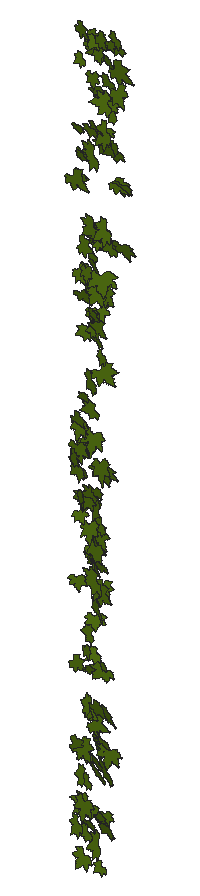
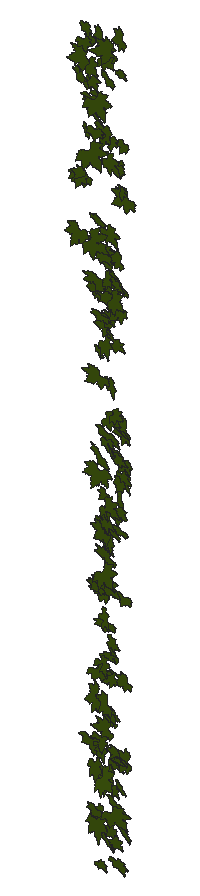
# SketchUp Ruby script. Lengths in inches.
U = 1.inch
M = Sketchup.active_model
def pt(a) = Geom::Point3d.new(a.map { |v| v * U })
def face(e, loops, mat)
  f = e.add_face(loops[0].map { |a| pt(a) })
  loops[1..].each { |l| e.add_face(l.map { |a| pt(a) }).erase! }
  f.material = f.back_material = mat if mat
  f
end
# faces: each face lists its corners as indices into pts; further lists are holes
def faces(e, pts, list, mat = nil) = list.each { |f| face(e, (f[0].is_a?(Array) ? f : [f]).map { |l| l.map { |i| pts[i] } }, mat) }
# xy, xz, yz: faces in a plane at the given z, y or x. An outline is a flat list of corners, or four numbers for a rectangle; further outlines are holes
def ring(l) = l.size == 4 ? [[l[0], l[1]], [l[2], l[1]], [l[2], l[3]], [l[0], l[3]]] : l.each_slice(2).to_a
def flat(e, list, mat, &to3) = list.each { |f| face(e, (f[0].is_a?(Array) ? f : [f]).map { |l| ring(l).map { |u, v| to3.(u, v) } }, mat) }
def xy(e, z, list, mat = nil) = flat(e, list, mat) { |x, y| [x, y, z] }
def xz(e, y, list, mat = nil) = flat(e, list, mat) { |x, z| [x, y, z] }
def yz(e, x, list, mat = nil) = flat(e, list, mat) { |y, z| [x, y, z] }
def lines(e, pts, list) = list.each { |a, b| e.add_line(pt(pts[a]), pt(pts[b])) }
# prism: a flat outline (further loops are holes) pulled along v
def prism(e, loops, v, mat = nil)
  f = face(e, loops, mat); d = Geom::Vector3d.new(v.map { |x| x * U })
  f.pushpull(f.normal.samedirection?(d) ? d.length : -d.length)
end
def box(e, o, s, mat = nil) = prism(e, [[o, [o[0] + s[0], o[1], o[2]], [o[0] + s[0], o[1] + s[1], o[2]], [o[0], o[1] + s[1], o[2]]]], [0, 0, s[2]], mat)
def at(x, y, z, deg = 0) = Geom::Transformation.translation(pt([x, y, z])) * Geom::Transformation.rotation(ORIGIN, Z_AXIS, deg.degrees)
def axes(o, x, y, z) = Geom::Transformation.new([*x, 0, *y, 0, *z, 0, *pt(o).to_a, 1])
def part(name) = M.definitions.add(name)
# library, detail: a bought-in or finely detailed component or shape, given as its bounding box
def library(name, o, s) = part(name).tap { |d| box(d.entities, o, s) }
def detail(e, o, s) = box(e.add_group.entities, o, s)
def put(e, d, t, mat = nil) = e.add_instance(d, t).tap { |i| i.material = mat if mat }
def group(e, t, mat = nil) = e.add_group.tap { |g| g.transformation = t; g.material = mat if mat }.entities
root = M.entities
M.materials.add("[Vegetation Blur 03]").color = [83, 114, 18]
c1 = part("ivy")
xy(c1.entities,0,[[0.782,0,0.786,0,0.787,0.005,0.789,0.009,0.821,0.072,0.875,0.147,1.001,0.272,1.073,0.331,1.137,0.363,1.178,0.379,1.223,0.384,1.272,0.383,1.311,0.374,1.36,0.355,1.399,0.334,1.491,0.285,1.541,0.244,1.583,0.199,1.617,0.15,1.64,0.128,1.662,0.115,1.717,0.105,1.745,0.093,1.784,0.054,1.819,0.057,1.854,0.064,1.882,0.075,1.896,0.074,1.91,0.071,1.937,0.063,1.964,0.053,1.99,0.038,2.016,0.015,2.034,0.002,2.04,0,2.038,0.003,2.036,0.007,2.033,0.038,2.036,0.068,2.045,0.1,2.055,0.116,2.064,0.123,2.077,0.129,2.088,0.129,2.106,0.132,2.118,0.13,2.179,0.132,2.207,0.133,2.225,0.133,2.242,0.138,2.22,0.162,2.207,0.186,2.206,0.213,2.212,0.236,2.228,0.262,2.247,0.274,2.298,0.283,2.355,0.294,2.37,0.296,2.376,0.295,2.377,0.3,2.377,0.303,2.385,0.329,2.411,0.37,2.426,0.392,2.449,0.407,2.511,0.426,2.561,0.444,2.619,0.466,2.589,0.469,2.561,0.476,2.501,0.5,2.449,0.516,2.424,0.523,2.401,0.535,2.377,0.556,2.372,0.568,2.36,0.575,2.268,0.586,2.225,0.592,2.207,0.599,2.194,0.61,2.143,0.65,2.13,0.664,2.122,0.682,2.123,0.7,2.13,0.719,2.148,0.75,2.17,0.781,2.195,0.807,2.221,0.828,2.284,0.874,2.291,0.88,2.288,0.887,2.276,0.9,2.267,0.916,2.265,0.933,2.273,0.967,2.292,1.002,2.313,1.03,2.334,1.054,2.348,1.067,2.358,1.074,2.363,1.076,2.362,1.081,2.35,1.094,2.347,1.11,2.35,1.143,2.359,1.18,2.385,1.254,2.415,1.324,2.448,1.393,2.45,1.4,2.446,1.398,2.44,1.394,2.427,1.383,2.402,1.36,2.376,1.339,2.345,1.324,2.305,1.309,2.282,1.303,2.273,1.306,2.245,1.294,2.212,1.287,2.187,1.291,2.163,1.301,2.142,1.316,2.134,1.327,2.124,1.325,2.09,1.292,2.053,1.259,2.014,1.234,1.973,1.215,1.954,1.21,1.931,1.208,1.909,1.212,1.893,1.22,1.879,1.233,1.872,1.248,1.867,1.281,1.864,1.319,1.821,1.258,1.773,1.197,1.726,1.141,1.698,1.121,1.679,1.116,1.666,1.117,1.647,1.122,1.632,1.129,1.62,1.141,1.617,1.154,1.617,1.219,1.621,1.254,1.623,1.268,1.623,1.281,1.618,1.314,1.606,1.346,1.603,1.375,1.607,1.403,1.603,1.467,1.599,1.499,1.605,1.525,1.614,1.552,1.629,1.577,1.635,1.589,1.629,1.587,1.618,1.582,1.596,1.566,1.581,1.556,1.568,1.552,1.557,1.55,1.545,1.553,1.531,1.562,1.522,1.572,1.504,1.591,1.486,1.611,1.474,1.631,1.457,1.666,1.455,1.684,1.457,1.698,1.452,1.715,1.444,1.728,1.424,1.754,1.419,1.772,1.423,1.786,1.434,1.819,1.444,1.848,1.446,1.855,1.44,1.861,1.43,1.867,1.386,1.904,1.349,1.948,1.326,1.973,1.31,1.995,1.288,2.048,1.284,2.153,1.287,2.254,1.284,2.255,1.282,2.253,1.278,2.247,1.274,2.237,1.266,2.216,1.226,2.125,1.208,2.076,1.184,2.033,1.155,1.984,1.135,1.942,1.111,1.899,1.083,1.861,1.053,1.85,1.059,1.83,1.061,1.809,1.056,1.79,1.049,1.767,1.04,1.749,1.018,1.733,0.994,1.726,0.942,1.734,0.95,1.6875,0.944,1.645,0.932,1.608,0.911,1.585,0.881,1.58,0.854,1.582,0.828,1.588,0.785,1.618,0.773,1.625,0.775,1.614,0.779,1.598,0.796,1.502,0.818,1.402,0.861,1.283,0.882,1.224,0.894,1.174,0.892,1.148,0.886,1.123,0.881,1.107,0.872,1.099,0.849,1.094,0.818,1.092,0.789,1.098,0.762,1.107,0.753,1.113,0.721,1.139,0.698,1.163,0.678,1.194,0.665,1.224,0.628,1.28,0.612,1.312,0.606,1.327,0.606,1.314,0.599,1.282,0.594,1.267,0.581,1.256,0.544,1.245,0.512,1.244,0.473,1.249,0.444,1.256,0.382,1.288,0.339,1.306,0.324,1.316,0.317,1.324,0.309,1.326,0.27,1.314,0.227,1.313,0.185,1.3125,0.152,1.317,0.122,1.328,0.092,1.345,0.073,1.353,0.079,1.338,0.092,1.308,0.117,1.249,0.13,1.215,0.139,1.164,0.147,1.148,0.157,1.136,0.163,1.122,0.174,1.086,0.177,1.067,0.182,1.054,0.186,1.043,0.191,1.038,0.211,1.028,0.237,1.005,0.25,0.974,0.253,0.96,0.25,0.944,0.242,0.914,0.243,0.906,0.249,0.902,0.26,0.894,0.289,0.88,0.307,0.873,0.322,0.862,0.364,0.799,0.403,0.738,0.431,0.709,0.439,0.691,0.441,0.678,0.4375,0.66,0.428,0.645,0.394,0.623,0.303,0.594,0.255,0.581,0.214,0.577,0.179,0.573,0.173,0.568,0.175,0.561,0.167,0.55,0.141,0.523,0.113,0.503,0.077,0.49,0.045,0.486,0.026,0.485,0.019,0.486,0.011,0.483,0,0.471,0.014,0.467,0.044,0.455,0.058,0.447,0.07,0.438,0.097,0.411,0.125,0.394,0.158,0.377,0.174,0.366,0.182,0.359,0.185,0.361,0.242,0.331,0.253,0.316,0.258,0.303,0.262,0.283,0.274,0.278,0.308,0.274,0.341,0.252,0.366,0.226,0.366,0.222,0.37,0.22,0.38,0.221,0.395,0.221,0.425,0.216,0.45,0.207,0.465,0.192,0.473,0.178,0.484,0.15,0.489,0.116,0.483,0.089,0.468,0.058,0.45,0.035,0.435,0.018,0.429,0.011,0.434,0.012,0.438,0.014,0.469,0.019,0.542,0.016,0.581,0.015,0.612,0.027,0.68,0.055,0.696,0.057,0.712,0.052,0.73,0.045,0.741,0.036,0.766,0.014]])
p = [[86.74,174.5,94.56],[86.66,174.5,94.56]]
lines(root,p,[[0,1]])
put(root,c1,axes([83.45,173.7,84.39],[0.11247,0.10768,-0.41349],[-0.50254,0.19726,-0.08297],[-0.08291,-1.04957,-0.05801]),"[Vegetation Blur 03]")
put(root,c1,axes([82.4,173.7,68.58],[0.38704,0.02073,0.09682],[0.11906,-0.06304,-0.31489],[0.00062,-0.83064,0.02631]),"[Vegetation Blur 03]")
put(root,c1,axes([82.79,173.7,75.08],[0.46711,-0.27655,-0.25561],[-0.31156,0.09667,-0.39569],[-0.13813,-1.15324,0.02812]),"[Vegetation Blur 03]")
put(root,c1,axes([82.6,173.7,91.86],[0.29162,-0.09248,0.04712],[0.06325,0.07335,-0.23812],[-0.03677,-0.60733,-0.03593]),"[Vegetation Blur 03]")
put(root,c1,axes([82.36,173.7,63.95],[0.20869,-0.00294,0.30527],[0.37402,-0.00987,-0.17032],[-0.00489,-0.88135,0.00089]),"[Vegetation Blur 03]")
put(root,c1,axes([82.53,173.7,74.5625],[0.11578,-0.07742,0.31422],[0.36947,-0.22297,-0.09932],[-0.11465,-0.79672,-0.00274]),"[Vegetation Blur 03]")
put(root,c1,axes([82.08,173.7,88.79],[0.38841,-0.03974,0.39058],[0.47889,0.01108,-0.31703],[-0.00798,-1.26829,-0.01501]),"[Vegetation Blur 03]")
put(root,c1,axes([82.88,173.7,89.65],[0.29613,-0.07388,-0.10232],[-0.12287,0.05638,-0.24327],[-0.04369,-0.65932,-0.00934]),"[Vegetation Blur 03]")
put(root,c1,axes([83.37,173.7,59.11],[0.14128,-0.20319,-0.29587],[-0.36071,0.14973,-0.1309],[-0.10517,-0.78653,0.05152]),"[Vegetation Blur 03]")
put(root,c1,axes([83.1,173.7,95.71],[0.23115,-0.1069,-0.165],[-0.20647,-0.0259,-0.19002],[-0.03067,-0.63139,0.03573]),"[Vegetation Blur 03]")
put(root,c1,axes([83.41,173.7,78.21],[0.08326,0.10722,-0.24971],[-0.31037,0.02564,-0.0672],[0.00148,-0.65202,-0.0437]),"[Vegetation Blur 03]")
put(root,c1,axes([82.8125,173.7,56.57],[0.42261,-0.28747,-0.1193],[-0.16204,-0.06467,-0.35783],[-0.12093,-0.91792,0.06257]),"[Vegetation Blur 03]")
put(root,c1,axes([82.48,173.7,59.61],[0.11289,-0.08937,0.40816],[0.50197,0.01041,-0.09212],[-0.00461,-1.05497,-0.03549]),"[Vegetation Blur 03]")
put(root,c1,axes([83.47,173.7,75.94],[0.13432,-0.12713,-0.31462],[-0.38869,0.03529,-0.11278],[-0.03669,-0.83931,0.04291]),"[Vegetation Blur 03]")
put(root,c1,axes([82.91,173.7,90.74],[0.29319,-0.08212,-0.05398],[-0.06371,0.04494,-0.24127],[-0.04367,-0.61685,-0.01039]),"[Vegetation Blur 03]")
put(root,c1,axes([82.6,173.7,71.81],[0.27283,0.0757,0.1916],[0.23721,-0.13013,-0.2169],[-0.01401,-0.72914,0.0586]),"[Vegetation Blur 03]")
put(root,c1,axes([82.38,173.7,75.48],[0.52424,-0.12738,0.15619],[0.18843,-0.07357,-0.4307],[-0.07036,-1.14606,0.01029]),"[Vegetation Blur 03]")
put(root,c1,axes([83.38,173.7,81.78],[0.19574,-0.01438,-0.25163],[-0.30815,-0.03945,-0.1593],[0.01245,-0.75048,0.0132]),"[Vegetation Blur 03]")
put(root,c1,axes([83.15,173.7,57.83],[0.47968,0.02946,-0.35016],[-0.4281,-0.06549,-0.39149],[0.03188,-1.32271,0.01158]),"[Vegetation Blur 03]")
put(root,c1,axes([83.65,173.7,84.9],[0.09556,-0.13792,-0.34176],[-0.41905,0.10501,-0.08471],[-0.06516,-0.87761,0.04357]),"[Vegetation Blur 03]")
put(root,c1,axes([82.79,173.7,74.375],[0.34163,-0.14558,0.05444],[0.07406,0.06471,-0.28235],[-0.063,-0.71335,-0.03672]),"[Vegetation Blur 03]")
put(root,c1,axes([82.59,173.7,84.14],[0.2559,0.03571,0.2999],[0.36108,-0.20047,-0.20147],[-0.07032,-0.89939,0.05682]),"[Vegetation Blur 03]")
put(root,c1,axes([83.25,173.7,60.26],[0.31122,-0.06083,-0.21678],[-0.26689,-0.02709,-0.25402],[-0.01391,-0.84152,0.02385]),"[Vegetation Blur 03]")
put(root,c1,axes([83.4,173.7,56.21],[0.24157,-0.07416,-0.2538],[-0.31175,0.01688,-0.19842],[-0.02861,-0.81014,0.0191]),"[Vegetation Blur 03]")
put(root,c1,axes([82.6,173.7,83.19],[0.40086,-0.0573,0.17483],[0.21594,0.13183,-0.32299],[0.00594,-0.92596,-0.0568]),"[Vegetation Blur 03]")
put(root,c1,axes([82.9,173.7,90.23],[0.11718,-0.12684,0.22641],[0.28293,-0.00575,-0.09804],[-0.02661,-0.61967,-0.04543]),"[Vegetation Blur 03]")
put(root,c1,axes([82.81,173.7,73.18],[0.52679,-0.06661,-0.07919],[-0.09633,0.02908,-0.43069],[-0.03439,-1.10187,-0.00658]),"[Vegetation Blur 03]")
put(root,c1,axes([82.7,173.7,76.92],[0.52102,-0.20474,0.04178],[0.03433,-0.18504,-0.42777],[-0.1065,-1.06132,0.06652]),"[Vegetation Blur 03]")
put(root,c1,axes([83.79,173.7,62.77],[0.05013,-0.17245,-0.31461],[-0.38087,0.18721,-0.05657],[-0.1028,-0.77773,0.05615]),"[Vegetation Blur 03]")
put(root,c1,axes([83,173.7,54.99],[0.48428,-0.17048,-0.13656],[-0.17611,-0.0992,-0.39652],[-0.06201,-1.04969,0.05965]),"[Vegetation Blur 03]")
put(root,c1,axes([82.49,173.7,76.59],[0.31137,-0.19726,0.4006],[0.48849,-0.13513,-0.26337],[-0.10722,-1.1885,-0.03655]),"[Vegetation Blur 03]")
put(root,c1,axes([83.89,173.7,59.78],[0.15704,0.2136,-0.46973],[-0.57168,0.3147,-0.1048],[-0.12334,-1.18664,-0.11235]),"[Vegetation Blur 03]")
put(root,c1,axes([83.49,173.7,58.8],[0.21308,-0.10262,-0.22404],[-0.27243,0.07685,-0.17812],[-0.0602,-0.71097,0.01308]),"[Vegetation Blur 03]")
put(root,c1,axes([83.8125,173.7,66.47],[0.09612,-0.08439,-0.33414],[-0.40558,0.12635,-0.08273],[-0.06933,-0.85613,0.02072]),"[Vegetation Blur 03]")
put(root,c1,axes([83.82,173.7,73.61],[0.20248,0.05039,-0.42079],[-0.51446,0.11243,-0.16277],[-0.042,-1.13431,-0.03483]),"[Vegetation Blur 03]")
put(root,c1,axes([82.9,173.7,85.32],[0.06821,0.02412,0.38984],[0.47536,-0.1037,-0.05439],[-0.04826,-0.98747,0.01524]),"[Vegetation Blur 03]")
put(root,c1,axes([82.76,173.7,96.75],[0.24867,-0.15858,0.33537],[0.40835,-0.11898,-0.21053],[-0.08971,-0.98119,-0.02867]),"[Vegetation Blur 03]")
put(root,c1,axes([83.82,173.7,77.97],[0.16222,0.03807,-0.33908],[-0.41557,-0.02093,-0.13279],[0.01621,-0.91758,-0.01104]),"[Vegetation Blur 03]")
put(root,c1,axes([82.57,173.7,59.83],[0.38921,-0.01895,0.37093],[0.44943,-0.16908,-0.31546],[-0.06835,-1.21968,0.03797]),"[Vegetation Blur 03]")
put(root,c1,axes([83.86,173.7,85.18],[0.08292,0.05054,-0.29306],[-0.34577,0.22171,-0.05915],[-0.09993,-0.72524,-0.0385]),"[Vegetation Blur 03]")
put(root,c1,axes([83.69,173.7,70.22],[0.33518,0.12814,-0.38098],[-0.46864,0.20726,-0.26366],[-0.04654,-1.16428,-0.08887]),"[Vegetation Blur 03]")
put(root,c1,axes([83.77,173.7,91.36],[0.33503,-0.17484,-0.44401],[-0.53885,0.1655,-0.28108],[-0.11328,-1.30432,0.02385]),"[Vegetation Blur 03]")
put(root,c1,axes([82.92,173.7,73.04],[0.31064,-0.27454,0.24989],[0.28954,-0.20759,-0.27561],[-0.1665,-0.87322,-0.01304]),"[Vegetation Blur 03]")
put(root,c1,axes([84.19,173.7,73.03],[0.10156,-0.07064,-0.4993],[-0.59327,0.30784,-0.08723],[-0.15326,-1.23847,0.0068]),"[Vegetation Blur 03]")
put(root,c1,axes([83.29,173.7,92.1],[0.37183,-0.05449,-0.06268],[-0.07386,0.08152,-0.30299],[-0.03383,-0.77703,-0.02739]),"[Vegetation Blur 03]")
put(root,c1,axes([83.92,173.7,69.5],[0.29364,-0.08887,-0.43973],[-0.53794,0.07502,-0.24166],[-0.05272,-1.26047,0.01662]),"[Vegetation Blur 03]")
put(root,c1,axes([83.3,173.7,61.67],[0.05383,0.00628,0.24765],[0.29967,-0.10102,-0.04299],[-0.04781,-0.62607,0.00942]),"[Vegetation Blur 03]")
put(root,c1,axes([83.78,173.7,86.52],[0.25146,0.10077,-0.27244],[-0.33679,0.12568,-0.19974],[-0.01997,-0.85077,-0.06178]),"[Vegetation Blur 03]")
put(root,c1,axes([83.6,173.7,87.57],[0.45075,-0.16208,-0.3284],[-0.40131,0.07789,-0.37294],[-0.08406,-1.24093,0.01948]),"[Vegetation Blur 03]")
put(root,c1,axes([82.9,173.7,57.62],[0.59208,-0.24793,0.06374],[0.06017,-0.19072,-0.48897],[-0.13036,-1.21404,0.0638]),"[Vegetation Blur 03]")
put(root,c1,axes([83.22,173.7,63.97],[0.19108,-0.09038,0.20852],[0.25839,0.11931,-0.14958],[0.021,-0.6456,-0.05683]),"[Vegetation Blur 03]")
put(root,c1,axes([83.13,173.7,84.73],[0.36627,-0.13941,0.12421],[0.13945,-0.15724,-0.30166],[-0.09113,-0.8009,0.0376]),"[Vegetation Blur 03]")
put(root,c1,axes([83.69,173.7,85.79],[0.23501,-0.07019,-0.1629],[-0.19555,0.08472,-0.19365],[-0.05258,-0.62881,-0.00791]),"[Vegetation Blur 03]")
put(root,c1,axes([83.2,173.7,65.14],[0.25479,-0.12423,0.18023],[0.21133,-0.13383,-0.2135],[-0.08804,-0.68079,0.00908]),"[Vegetation Blur 03]")
put(root,c1,axes([83.62,173.7,71.66],[0.37161,-0.21861,-0.25288],[-0.28876,0.23657,-0.31481],[-0.15463,-0.96714,-0.01984]),"[Vegetation Blur 03]")
put(root,c1,axes([83.25,173.7,56.28],[0.2775,-0.12673,0.11481],[0.14869,0.07236,-0.22682],[-0.03837,-0.63611,-0.04867]),"[Vegetation Blur 03]")
put(root,c1,axes([83.95,173.7,96.4],[0.21316,0.03069,-0.31446],[-0.38542,0.04396,-0.17335],[-0.01149,-0.90506,-0.01908]),"[Vegetation Blur 03]")
put(root,c1,axes([83.87,173.7,82.06],[0.16581,-0.12598,-0.20066],[-0.24842,0.03821,-0.1405],[-0.04988,-0.60905,0.03269]),"[Vegetation Blur 03]")
put(root,c1,axes([84.05,173.7,67.84],[0.20676,-0.07941,-0.38547],[-0.44776,0.31453,-0.17016],[-0.15519,-1.01328,-0.02261]),"[Vegetation Blur 03]")
put(root,c1,axes([83.78,173.7,81.8],[0.3273,-0.0909,-0.29956],[-0.34726,0.27044,-0.26563],[-0.12681,-0.97518,-0.04574]),"[Vegetation Blur 03]")
put(root,c1,axes([83.56,173.7,79.63],[0.43303,-0.27941,-0.22313],[-0.26455,0.14367,-0.37028],[-0.1523,-1.044,0.00876]),"[Vegetation Blur 03]")
put(root,c1,axes([83.47,173.7,59.71],[0.5589,-0.19272,-0.25961],[-0.28238,0.39595,-0.45114],[-0.17385,-1.26271,-0.10184]),"[Vegetation Blur 03]")
put(root,c1,axes([83.56,173.7,76.42],[0.33014,-0.06379,-0.05513],[-0.06679,0.02302,-0.2706],[-0.03261,-0.69306,-0.00391]),"[Vegetation Blur 03]")
put(root,c1,axes([83.44,173.7,61.71],[0.13106,0.04715,0.22271],[0.27208,-0.09295,-0.10355],[-0.03102,-0.61597,0.03267]),"[Vegetation Blur 03]")
put(root,c1,axes([83.42,173.7,82.65],[0.34203,-0.05341,0.04309],[0.05121,-0.04542,-0.27956],[-0.02898,-0.71072,0.01463]),"[Vegetation Blur 03]")
put(root,c1,axes([83.64,173.7,96.8125],[0.33694,0.0048,-0.1079],[-0.13035,-0.11296,-0.27192],[0.0222,-0.7362,0.04102]),"[Vegetation Blur 03]")
put(root,c1,axes([83.44,173.7,75.48],[0.09035,0.0602,0.28294],[0.33236,-0.23291,-0.06289],[-0.10289,-0.69949,0.04529]),"[Vegetation Blur 03]")
put(root,c1,axes([83.89,173.7,65.49],[0.26178,-0.07777,-0.19292],[-0.23918,-0.11506,-0.20887],[0.01,-0.71663,0.05447]),"[Vegetation Blur 03]")
put(root,c1,axes([83.14,173.7,71.55],[0.46252,-0.08041,0.20679],[0.23593,-0.28736,-0.36906],[-0.10033,-1.0465,0.08545]),"[Vegetation Blur 03]")
put(root,c1,axes([83.35,173.7,66.91],[0.41222,0.08825,0.09854],[0.12607,-0.1297,-0.333],[0.02291,-0.87434,0.05934]),"[Vegetation Blur 03]")
put(root,c1,axes([83.25,173.7,69.91],[0.09143,0.21564,0.47102],[0.58317,-0.16267,-0.06368],[-0.06308,-1.19139,0.09395]),"[Vegetation Blur 03]")
put(root,c1,axes([83.94,173.7,65.27],[0.3587,-0.08547,-0.26789],[-0.31864,0.17898,-0.29317],[-0.08908,-0.98439,-0.03004]),"[Vegetation Blur 03]")
put(root,c1,axes([83.69,173.7,84.04],[0.46854,-0.05722,-0.15501],[-0.19159,-0.07548,-0.38134],[-0.0119,-1.03762,0.03629]),"[Vegetation Blur 03]")
put(root,c1,axes([84.02,173.7,60.8],[0.31159,-0.10577,-0.25159],[-0.29051,0.23223,-0.255],[-0.11522,-0.87155,-0.03742]),"[Vegetation Blur 03]")
put(root,c1,axes([83.44,173.7,94.8],[0.3823,-0.12513,0.1329],[0.15394,-0.13225,-0.31454],[-0.08072,-0.8448,0.02956]),"[Vegetation Blur 03]")
put(root,c1,axes([83.24,173.7,95.86],[0.15219,-0.0035,0.49259],[0.60198,0.09401,-0.12377],[0.04388,-1.27745,-0.01046]),"[Vegetation Blur 03]")
put(root,c1,axes([83.59,173.7,82.125],[0.08947,-0.09548,0.30203],[0.3696,-0.08246,-0.07703],[-0.05008,-0.77914,-0.02886]),"[Vegetation Blur 03]")
put(root,c1,axes([84.17,173.7,56.15],[0.33567,-0.36714,-0.32626],[-0.40941,0.10373,-0.29893],[-0.15499,-1.06915,0.08303]),"[Vegetation Blur 03]")
put(root,c1,axes([83.98,173.7,94.33],[0.49914,0.06889,-0.35402],[-0.43405,0.1716,-0.40237],[-0.0297,-1.34994,-0.06922]),"[Vegetation Blur 03]")
put(root,c1,axes([83.26,173.7,76.58],[0.64177,-0.16774,0.0763],[0.07979,-0.21804,-0.52237],[-0.09498,-1.31665,0.07678]),"[Vegetation Blur 03]")
put(root,c1,axes([84.62,173.7,87.19],[0.20681,0.14961,-0.50522],[-0.62308,0.08477,-0.16594],[-0.01632,-1.34039,-0.06689]),"[Vegetation Blur 03]")
put(root,c1,axes([83.7,173.7,73.4],[0.23912,-0.07387,0.13682],[0.16931,0.00875,-0.19635],[-0.02693,-0.60087,-0.01968]),"[Vegetation Blur 03]")
put(root,c1,axes([83.46,173.7,60.95],[0.10403,0.04174,0.45584],[0.55849,-0.05312,-0.08413],[-0.02168,-1.16792,0.02012]),"[Vegetation Blur 03]")
put(root,c1,axes([84.01,173.7,64.82],[0.41939,0.05909,-0.24373],[-0.29711,-0.06483,-0.343],[0.04165,-1.05748,0.00741]),"[Vegetation Blur 03]")
put(root,c1,axes([83.6875,173.7,85.9],[0.15956,0.10306,0.24419],[0.30313,-0.02658,-0.13017],[0.01203,-0.69728,0.04105]),"[Vegetation Blur 03]")
put(root,c1,axes([83.6,173.7,92.42],[0.59182,-0.28218,-0.07799],[-0.07654,0.18572,-0.49252],[-0.14859,-1.21956,-0.05695]),"[Vegetation Blur 03]")
put(root,c1,axes([84.18,173.7,54.625],[0.26116,-0.07939,-0.16142],[-0.20062,-0.0401,-0.21311],[-0.01886,-0.67295,0.03174]),"[Vegetation Blur 03]")
put(root,c1,axes([83.9,173.7,61.1875],[0.45644,-0.12973,-0.15733],[-0.18474,0.13729,-0.3748],[-0.08372,-1.01031,-0.03073]),"[Vegetation Blur 03]")
put(root,c1,axes([83.61,173.7,82.54],[0.32504,0.10399,0.20827],[0.26014,-0.12611,-0.26052],[0.00118,-0.84097,0.06482]),"[Vegetation Blur 03]")
put(root,c1,axes([84.35,173.7,91.73],[0.44413,0.17265,-0.41061],[-0.51006,0.15289,-0.35736],[-0.00095,-1.3725,-0.09146]),"[Vegetation Blur 03]")
put(root,c1,axes([83.96,173.7,57.05],[0.5663,-0.16171,-0.26651],[-0.30497,0.30432,-0.46069],[-0.14072,-1.31032,-0.0741]),"[Vegetation Blur 03]")
put(root,c1,axes([84.1875,173.7,72.29],[0.32555,-0.21056,-0.17248],[-0.21105,0.06347,-0.27751],[-0.10292,-0.79617,0.02349]),"[Vegetation Blur 03]")
put(root,c1,axes([83.5,173.7,62.29],[0.35259,-0.1904,0.31199],[0.38853,0.00444,-0.29204],[-0.06112,-1.07015,-0.05672]),"[Vegetation Blur 03]")
put(root,c1,axes([84.82,173.7,94.18],[0.12519,-0.10736,-0.42184],[-0.51949,-0.03465,-0.1013],[0.00417,-1.09384,0.04461]),"[Vegetation Blur 03]")
put(root,c1,axes([83.81,173.7,95.92],[0.26564,-0.06538,0.20861],[0.24422,-0.17627,-0.21582],[-0.08188,-0.73784,0.03307]),"[Vegetation Blur 03]")
put(root,c1,axes([83.58,173.7,70.9],[0.57824,-0.2854,0.09144],[0.09076,-0.20234,-0.48162],[-0.15346,-1.19504,0.05971]),"[Vegetation Blur 03]")
put(root,c1,axes([83.4,173.7,84.52],[0.63449,0.08244,0.15008],[0.18708,-0.13099,-0.51549],[0.02055,-1.35306,0.05905]),"[Vegetation Blur 03]")
put(root,c1,axes([84.7,173.7,95.91],[0.1485,0.06744,-0.32773],[-0.39216,0.22625,-0.11103],[-0.09244,-0.8515,-0.05546]),"[Vegetation Blur 03]")
put(root,c1,axes([83.59,173.7,81.63],[0.21618,-0.06557,0.43271],[0.52184,-0.19331,-0.17826],[-0.09899,-1.16227,0.00524]),"[Vegetation Blur 03]")
put(root,c1,axes([83.5,173.7,74.7],[0.61927,-0.03223,0.11526],[0.14207,0.12094,-0.50313],[-0.00213,-1.30144,-0.04961]),"[Vegetation Blur 03]")
put(root,c1,axes([83.4,173.7,71.15],[0.45704,-0.07073,0.34791],[0.42202,-0.13355,-0.37354],[-0.06933,-1.27915,0.01976]),"[Vegetation Blur 03]")
put(root,c1,axes([84.24,173.7,59.85],[0.48214,-0.22782,-0.28181],[-0.31501,0.32234,-0.39997],[-0.17959,-1.177,-0.05499]),"[Vegetation Blur 03]")
put(root,c1,axes([83.71,173.7,69.76],[0.23423,-0.31556,0.37462],[0.44905,-0.24958,-0.22008],[-0.18046,-1.03065,-0.06141]),"[Vegetation Blur 03]")
put(root,c1,axes([83.9375,173.7,56.6875],[0.21432,-0.13844,0.2244],[0.28013,0.00181,-0.17803],[-0.04065,-0.71738,-0.04375]),"[Vegetation Blur 03]")
put(root,c1,axes([83.56,173.7,79.27],[0.38223,0.09975,0.36551],[0.44923,0.00523,-0.31313],[0.03341,-1.2116,0.02874]),"[Vegetation Blur 03]")
put(root,c1,axes([84.18,173.7,80.8125],[0.32645,-0.19251,-0.02516],[-0.03795,-0.04316,-0.27603],[-0.0909,-0.67338,0.02489]),"[Vegetation Blur 03]")
put(root,c1,axes([84.0625,173.7,92.17],[0.36239,0.03439,0.0325],[0.04011,-0.01114,-0.29602],[0.01602,-0.75014,0.00588]),"[Vegetation Blur 03]")
put(root,c1,axes([84.5,173.7,95.07],[0.31224,-0.04153,-0.22289],[-0.2695,0.10455,-0.25454],[-0.04857,-0.84719,-0.02048]),"[Vegetation Blur 03]")
put(root,c1,axes([83.72,173.7,67.93],[0.19345,-0.03327,0.47278],[0.57353,-0.16922,-0.15818],[-0.0831,-1.24533,0.00886]),"[Vegetation Blur 03]")
put(root,c1,axes([83.92,173.7,96.58],[0.22749,-0.09368,0.31124],[0.37139,-0.17878,-0.18927],[-0.09787,-0.89612,0.00522]),"[Vegetation Blur 03]")
put(root,c1,axes([83.9,173.7,68.41],[0.30062,0.06409,0.25513],[0.31279,-0.14376,-0.23982],[-0.02918,-0.88082,0.05771]),"[Vegetation Blur 03]")
put(root,c1,axes([84.76,173.7,86.62],[0.2286,-0.00259,-0.27195],[-0.33307,0.02295,-0.18652],[-0.00991,-0.83122,-0.0043]),"[Vegetation Blur 03]")
put(root,c1,axes([84.47,173.7,87.75],[0.44457,-0.30415,-0.24459],[-0.31847,-0.07486,-0.37092],[-0.10118,-1.10076,0.09281]),"[Vegetation Blur 03]")
put(root,c1,axes([84.11,173.7,56.98],[0.33883,-0.03876,0.14234],[0.17237,-0.07132,-0.27636],[-0.03256,-0.78094,0.01817]),"[Vegetation Blur 03]")
put(root,c1,axes([83.76,173.7,74.98],[0.53293,-0.19106,0.2627],[0.2994,-0.28671,-0.43737],[-0.15029,-1.24869,0.06023]),"[Vegetation Blur 03]")
put(root,c1,axes([84.49,173.7,92.81],[0.4979,-0.40473,-0.18477],[-0.2554,-0.09899,-0.42431],[-0.15719,-1.12116,0.10416]),"[Vegetation Blur 03]")
put(root,c1,axes([85.19,173.7,93.72],[0.11758,-0.14394,-0.33997],[-0.41694,0.10295,-0.1029],[-0.06765,-0.88473,0.04334]),"[Vegetation Blur 03]")
put(root,c1,axes([84.32,173.7,93.8],[0.42779,-0.01722,0.00276],[0.0027,-0.07154,-0.34805],[-0.00862,-0.87743,0.02832]),"[Vegetation Blur 03]")
put(root,c1,axes([84.2,173.7,83.4],[0.18898,0.02634,0.37085],[0.44381,-0.22984,-0.14807],[-0.09838,-0.98629,0.04441]),"[Vegetation Blur 03]")
put(root,c1,axes([84.14,173.7,60.68],[0.62343,-0.11777,0.0104],[0.0079,-0.1089,-0.50918],[-0.0581,-1.27854,0.04241]),"[Vegetation Blur 03]")
put(root,c1,axes([84.49,173.7,96.62],[0.24814,-0.07421,0.13501],[0.16554,-0.02052,-0.20443],[-0.03556,-0.61336,-0.0095]),"[Vegetation Blur 03]")
put(root,c1,axes([84.84,173.7,96.75],[0.32819,0.01887,-0.10221],[-0.12554,0.06541,-0.2666],[-0.0028,-0.71988,-0.0269]),"[Vegetation Blur 03]")
put(root,c1,axes([84.25,173.7,62.26],[0.31828,-0.32105,0.3684],[0.45752,-0.11523,-0.27908],[-0.137,-1.13071,-0.07616]),"[Vegetation Blur 03]")
put(root,c1,axes([84.91,173.7,97.43],[0.36865,-0.17556,-0.1237],[-0.14943,0.05438,-0.30876],[-0.08901,-0.81841,0.00602]),"[Vegetation Blur 03]")
put(root,c1,axes([84.87,173.7,91.74],[0.30667,-0.21087,0.08542],[0.09735,-0.07998,-0.26385],[-0.10945,-0.662,0.00467]),"[Vegetation Blur 03]")
put(root,c1,axes([84.61,173.7,89.29],[0.29759,0.01634,0.29239],[0.3571,0.0663,-0.24267],[0.02985,-0.95609,-0.01183]),"[Vegetation Blur 03]")
put(root,c1,axes([84.92,173.7,89.7],[0.43208,-0.00485,-0.01137],[-0.01346,0.125,-0.34915],[-0.00429,-0.88078,-0.04949]),"[Vegetation Blur 03]")
put(root,c1,axes([84.71,173.7,94.17],[0.38148,-0.02964,0.33346],[0.3977,-0.23961,-0.3064],[-0.09475,-1.12505,0.05647]),"[Vegetation Blur 03]")
put(root,c1,axes([84.8125,173.7,86.58],[0.54527,-0.10858,0.11727],[0.14945,0.14116,-0.4423],[-0.03309,-1.15173,-0.06527]),"[Vegetation Blur 03]")
put(root,c1,axes([84.65,173.7,95.01],[0.28018,-0.09633,0.48866],[0.59963,-0.03141,-0.22997],[-0.03369,-1.35996,-0.0293]),"[Vegetation Blur 03]")
